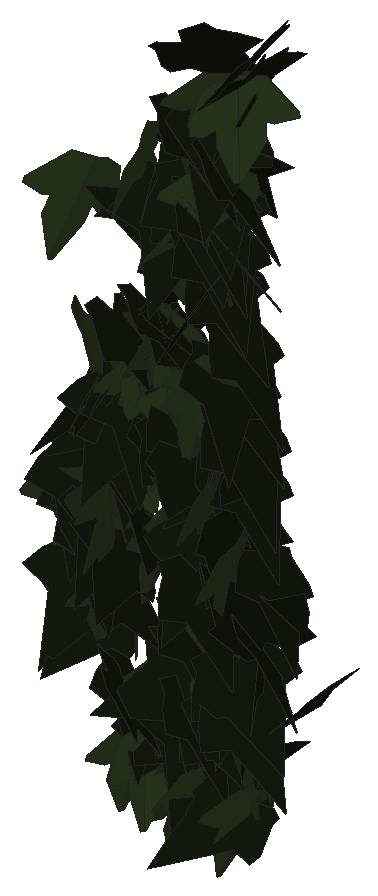
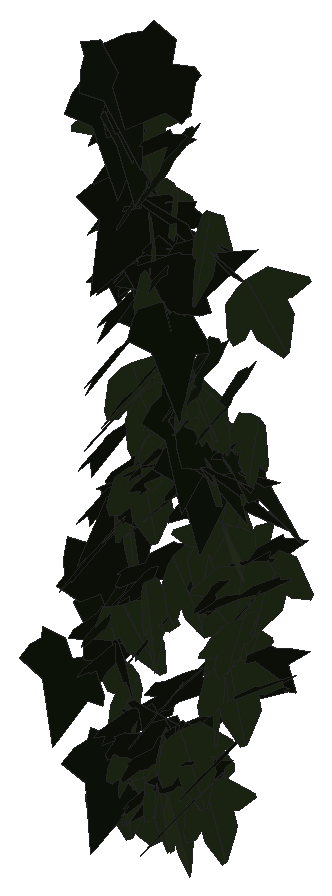
# SketchUp Ruby script. Lengths in inches.
U = 1.inch
M = Sketchup.active_model
def pt(a) = Geom::Point3d.new(a.map { |v| v * U })
def face(e, loops, mat)
  f = e.add_face(loops[0].map { |a| pt(a) })
  loops[1..].each { |l| e.add_face(l.map { |a| pt(a) }).erase! }
  f.material = f.back_material = mat if mat
  f
end
# faces: each face lists its corners as indices into pts; further lists are holes
def faces(e, pts, list, mat = nil) = list.each { |f| face(e, (f[0].is_a?(Array) ? f : [f]).map { |l| l.map { |i| pts[i] } }, mat) }
# xy, xz, yz: faces in a plane at the given z, y or x. An outline is a flat list of corners, or four numbers for a rectangle; further outlines are holes
def ring(l) = l.size == 4 ? [[l[0], l[1]], [l[2], l[1]], [l[2], l[3]], [l[0], l[3]]] : l.each_slice(2).to_a
def flat(e, list, mat, &to3) = list.each { |f| face(e, (f[0].is_a?(Array) ? f : [f]).map { |l| ring(l).map { |u, v| to3.(u, v) } }, mat) }
def xy(e, z, list, mat = nil) = flat(e, list, mat) { |x, y| [x, y, z] }
def xz(e, y, list, mat = nil) = flat(e, list, mat) { |x, z| [x, y, z] }
def yz(e, x, list, mat = nil) = flat(e, list, mat) { |y, z| [x, y, z] }
def lines(e, pts, list) = list.each { |a, b| e.add_line(pt(pts[a]), pt(pts[b])) }
# prism: a flat outline (further loops are holes) pulled along v
def prism(e, loops, v, mat = nil)
  f = face(e, loops, mat); d = Geom::Vector3d.new(v.map { |x| x * U })
  f.pushpull(f.normal.samedirection?(d) ? d.length : -d.length)
end
def box(e, o, s, mat = nil) = prism(e, [[o, [o[0] + s[0], o[1], o[2]], [o[0] + s[0], o[1] + s[1], o[2]], [o[0], o[1] + s[1], o[2]]]], [0, 0, s[2]], mat)
def at(x, y, z, deg = 0) = Geom::Transformation.translation(pt([x, y, z])) * Geom::Transformation.rotation(ORIGIN, Z_AXIS, deg.degrees)
def axes(o, x, y, z) = Geom::Transformation.new([*x, 0, *y, 0, *z, 0, *pt(o).to_a, 1])
def part(name) = M.definitions.add(name)
# library, detail: a bought-in or finely detailed component or shape, given as its bounding box
def library(name, o, s) = part(name).tap { |d| box(d.entities, o, s) }
def detail(e, o, s) = box(e.add_group.entities, o, s)
def put(e, d, t, mat = nil) = e.add_instance(d, t).tap { |i| i.material = mat if mat }
def group(e, t, mat = nil) = e.add_group.tap { |g| g.transformation = t; g.material = mat if mat }.entities
root = M.entities
M.materials.add("efeu1").color = [18, 25, 13]
M.materials.add("efeu2").color = [43, 57, 29]
c1 = part("ivyleaf_10")
p = [[0,0.5,-0.03],[-0.0625,2.02,-0.43],[-0.19,2.01,-0.46],[-0.54,1.05,-0.29],[-0.52,0.625,-0.18],[-0.83,0.76,-0.28],
  [-1.16,0.64,-0.33],[-1.15,0.33,-0.24],[-0.77,-0.39,0.02],[-0.3,-0.51,0.16],[0.04,-0.48,0.23],[-0.02,2.01,-0.4375],
  [-0.06,2.01,-0.43],[0.04,-0.49,0.23],[0.67,-0.49,0.14],[1.38,0.36,-0.2],[1.375,0.51,-0.24],[0.81,0.65,-0.19],
  [0.62,0.59,-0.15],[0.6,1.09,-0.28],[0.5,1.23,-0.31]]
faces(c1.entities,p,[[0,1,2,3,4,5,6,7,8,9,10],[11,12,0,13,14,15,16,17,18,19,20]],"efeu2")
c2 = part("ivyleaf_9")
p = [[1.54,2.16,1.25],[1.36,2.04,1.19],[-0.21,0.99,0.68],[-0.71,1.11,0.82],[-0.85,0.86,0.67],[-0.8,0.17,0.21],
  [-0.9,-0.01,0.1],[-0.67,-0.16,-0.02],[-0.08,-0.08,-0.05],[-0.03,-0.6,-0.4],[0.65,-0.88,-0.66],[0.83,-0.6,-0.49],
  [1.29,-0.42,-0.43],[1.8125,-0.07,-0.26],[1.21,0.44,0.15]]
faces(c2.entities,p,[[0,1,2,3,4,5,6,7,8,9,10,11,12,13,14]],"efeu1")
put(root,c1,axes([515.29,133.45,212.8],[-0.80305,-0.32335,-0.1119],[0.10212,0.04596,-0.8657],[0.32657,-0.80951,-0.00446]))
put(root,c2,axes([515.36,134.21,210.39],[-0.48603,-0.68308,0.11872],[-0.0493,-0.11057,-0.83801],[0.69156,-0.48795,0.0237]))
put(root,c1,axes([515.48,134.64,210.09],[-0.50146,-0.66753,0.15686],[-0.03057,-0.17238,-0.83128],[0.68503,-0.49635,0.07774]))
put(root,c2,axes([515.47,134.48,209.53],[-0.48983,-0.60352,0.33809],[-0.01133,-0.40721,-0.74332],[0.69167,-0.43407,0.22725]))
put(root,c1,axes([515.59,133.73,216.51],[-0.77942,0.38853,0.11578],[-0.12296,0.01252,-0.86982],[-0.38632,-0.78787,0.04327]))
put(root,c1,axes([515.375,134.55,211.5],[0.04627,0.85295,0.0692],[0.00684,0.06893,-0.8542],[-0.85573,0.04668,-0.00308]))
put(root,c1,axes([515.65,133.52,220.26],[-0.36653,-0.77477,0.4371],[-0.01066,-0.46889,-0.84006],[0.8895,-0.32487,0.17005]))
put(root,c2,axes([515.51,133.89,213.1],[-0.20454,-0.85126,0.02522],[-0.02053,-0.021,-0.87536],[0.85138,-0.20501,-0.01505]))
put(root,c2,axes([515.38,134.375,212.44],[-0.17335,-0.84195,-0.0494],[0.19386,0.0093,-0.83887],[0.82082,-0.18001,0.18769]))
put(root,c1,axes([515.53,134.25,212.82],[0.47061,0.7276,0.02766],[0.02328,0.01788,-0.86647],[-0.72775,0.47108,-0.00984]))
put(root,c2,axes([516.15,133.43,215.49],[-0.68936,0.51075,-0.19193],[0.10035,-0.1853,-0.85353],[-0.53631,-0.69117,0.087]))
put(root,c2,axes([515.67,134.29,212.7],[-0.0531,-0.86174,-0.09082],[-0.00711,0.09142,-0.86328],[0.86648,-0.05206,-0.01265]))
put(root,c1,axes([515.81,134.27,213.91],[0.46626,-0.59261,0.43719],[0.25158,-0.35815,-0.75376],[0.69212,0.5294,-0.02054]))
put(root,c1,axes([516.09,133.84,211.84],[-0.38547,-0.74939,0.19121],[0.03336,-0.22955,-0.83242],[0.77268,-0.36394,0.13133]))
put(root,c1,axes([516.12,133.97,210.58],[-0.15472,-0.8501,0.0923],[0.00598,-0.09487,-0.86376],[0.85507,-0.15316,0.02274]))
put(root,c2,axes([515.68,133.78,211.75],[0.20571,-0.83275,0.17944],[0.05578,-0.17104,-0.85769],[0.85004,0.21275,0.01286]))
put(root,c1,axes([516.22,134.57,206.42],[-0.24298,-0.78326,0.17958],[0.02267,-0.19422,-0.81642],[0.80326,-0.23145,0.07737]))
put(root,c2,axes([516.02,134.07,212.05],[-0.16234,-0.77343,0.35448],[-0.08781,-0.34372,-0.79016],[0.84625,-0.18403,-0.01399]))
put(root,c2,axes([516.62,134.21,215.09],[-0.84849,-0.07755,0.17646],[-0.16949,-0.07912,-0.84976],[0.09178,-0.86302,0.06205]))
put(root,c1,axes([516.28,134.3,209.93],[0.59117,-0.52975,-0.34968],[-0.08315,0.40909,-0.76035],[0.62928,0.55173,0.22802]))
put(root,c1,axes([516.12,133.52,212.74],[-0.16495,-0.8864,0.06493],[0.05275,0.05616,0.90066],[-0.88721,0.16814,0.04148]))
put(root,c1,axes([516.35,133.73,213.03],[-0.04646,-0.86798,-0.1242],[0.02358,0.12309,-0.86906],[0.8765,-0.04932,0.0168]))
put(root,c2,axes([515.96,134.84,207.62],[0.08172,-0.80698,0.22827],[0.0599,-0.22315,-0.81032],[0.83651,0.09481,0.03572]))
put(root,c1,axes([516.02,134.27,213.74],[0.56721,0.5549,0.35523],[0.20443,0.29737,-0.79095],[-0.62634,0.59956,0.06353]))
put(root,c1,axes([516.64,134.98,207.98],[-0.2977,-0.75396,0.19789],[-0.04916,-0.19325,-0.81024],[0.77795,-0.30073,0.02453]))
put(root,c2,axes([516.1,133.67,210.76],[0.57004,-0.55363,-0.32653],[-0.08496,0.36772,-0.77178],[0.63711,0.54438,0.18924]))
put(root,c2,axes([516.54,134.05,214.97],[-0.59831,-0.64533,0.00139],[0.09856,-0.09325,-0.8695],[0.63776,-0.591,0.13567]))
put(root,c2,axes([516.76,134.01,215.67],[0.11074,0.8712,0.03362],[-0.04947,0.04011,-0.87654],[-0.87044,0.10856,0.0541]))
put(root,c1,axes([516.6,132.95,212.625],[0.25317,-0.7476,-0.35306],[0.03552,0.37874,-0.77649],[0.82601,0.21285,0.1416]))
put(root,c2,axes([517.07,133.92,216.2],[-0.46371,0.74719,-0.10557],[-0.03048,-0.14235,-0.87365],[-0.754,-0.45377,0.10024]))
put(root,c2,axes([516.42,133.8,211.54],[-0.11313,-0.71017,0.49254],[0.07603,-0.50299,-0.70778],[0.8609,-0.0489,0.12723]))
put(root,c2,axes([516.32,135.09,206.64],[0.45394,-0.64181,-0.28018],[-0.04513,0.30638,-0.77497],[0.69885,0.43668,0.13194]))
put(root,c2,axes([516.58,134.11,214.71],[-0.25694,-0.83225,-0.11632],[0.01361,0.1175,-0.87074],[0.84023,-0.2564,-0.02147]))
put(root,c1,axes([516.77,134.14,215.33],[0.68092,-0.5423,-0.10008],[0.00844,0.16925,-0.85968],[0.55139,0.6671,0.13676]))
put(root,c1,axes([516.88,135.11,206.14],[0.22275,-0.79275,0.05545],[0.00747,-0.05549,-0.82341],[0.79465,0.22274,-0.0078]))
put(root,c2,axes([516.45,133.54,217.14],[0.55026,-0.69072,-0.10987],[-0.01035,0.13173,-0.88005],[0.69932,0.54544,0.07342]))
put(root,c1,axes([517.03,133.93,215.96],[-0.28301,-0.82945,0.11986],[0.01356,-0.13103,-0.87469],[0.83795,-0.27801,0.05464]))
put(root,c2,axes([516.78,134.05,215.3125],[-0.10439,-0.87209,-0.07403],[-0.00089,0.07466,-0.87827],[0.87523,-0.10394,-0.00972]))
put(root,c1,axes([516.92,133.97,206.73],[0.27693,0.80701,-0.11706],[-0.03925,-0.11029,-0.8532],[-0.81451,0.2797,0.00132]))
put(root,c2,axes([516.84,132.89,208.9],[0.73763,-0.27403,-0.46755],[-0.41717,0.21694,-0.7853],[0.34592,0.84596,0.04993]))
put(root,c2,axes([516.68,134.62,207.18],[0.25042,-0.57612,-0.54841],[0.09373,0.59232,-0.57945],[0.78987,0.11237,0.24263]))
put(root,c2,axes([517.35,133.84,216.47],[0.05893,0.86877,0.1688],[-0.02305,0.17062,-0.87011],[-0.88472,0.05342,0.03392]))
put(root,c1,axes([516.98,134.03,216.87],[-0.81277,-0.06604,-0.34802],[0.3473,0.02289,-0.81543],[0.06973,-0.88385,0.00488]))
put(root,c1,axes([517.23,133.76,216.83],[0.64335,-0.61121,-0.06337],[-0.03909,0.05086,-0.88734],[0.61324,0.64446,0.00993]))
put(root,c1,axes([517.09,133.74,216.06],[0.10849,0.81259,0.30422],[0.00524,0.30597,-0.81913],[-0.86765,0.10345,0.03309]))
put(root,c1,axes([517.28,133.27,221.38],[0.11171,-0.75215,-0.48219],[0.04222,0.48985,-0.75431],[0.89244,0.07097,0.09604]))
put(root,c1,axes([517.36,133.89,216.82],[0.09028,-0.88256,-0.05683],[-0.00008,0.05711,-0.88715],[0.88439,0.0901,0.00572]))
put(root,c1,axes([517.38,135.04,206.71],[0.01897,-0.82787,-0.03557],[0.001,0.0356,-0.82808],[0.82863,0.01891,0.00182]))
put(root,c1,axes([517.39,134.21,212.22],[0.07246,-0.88468,0.28141],[0.04261,-0.2788,-0.88744],[0.92738,0.08193,0.01878]))
put(root,c1,axes([518.02,133.34,215.7],[-0.1355,0.04894,0.8868],[-0.88801,-0.02342,-0.1344],[0.01579,-0.89678,0.0519]))
put(root,c2,axes([517.03,133.81,212.44],[0.04072,-0.56712,0.6413],[0.23385,-0.61024,-0.5545],[0.82354,0.20132,0.12575]))
put(root,c1,axes([517.51,133.84,217.11],[-0.51025,0.72885,0.03261],[-0.08067,-0.01682,-0.88648],[-0.7251,-0.51101,0.07568]))
put(root,c1,axes([517.54,134.57,207.53],[0.20361,-0.72912,-0.36426],[0.06412,0.38862,-0.74203],[0.81252,0.15204,0.14984]))
put(root,c2,axes([518.02,134.26,208.63],[-0.55301,-0.29719,0.58866],[-0.37205,-0.49369,-0.59876],[0.54445,-0.63923,0.18875]))
put(root,c2,axes([517.18,133.76,217.55],[0.55765,-0.68675,0.12788],[0.15763,-0.0357,-0.8791],[0.68053,0.57101,0.09883]))
put(root,c2,axes([518.4,133.73,219.6],[-0.08013,-0.00309,0.89127],[-0.88737,-0.08346,-0.08007],[0.0834,-0.89097,0.00441]))
put(root,c2,axes([517.43,133.69,214.77],[0.6087,-0.52528,-0.38295],[-0.10914,0.43459,-0.76961],[0.64082,0.57297,0.23267]))
put(root,c2,axes([518.17,133.69,218.83],[-0.12584,0.88894,0.02665],[-0.00201,0.02663,-0.8978],[-0.88933,-0.12584,-0.00174]))
put(root,c2,axes([517.59,134.66,206.68],[0.41321,-0.65407,-0.35834],[-0.02382,0.39788,-0.75371],[0.74542,0.37529,0.17455]))
put(root,c2,axes([518.52,134.36,207.91],[-0.82548,0.08718,0.2087],[-0.2107,-0.00937,-0.82951],[-0.0822,-0.8514,0.0305]))
put(root,c2,axes([517.84,134.71,207.41],[-0.17681,-0.86487,0.23013],[-0.03363,-0.22799,-0.88267],[0.89433,-0.17956,0.0123]))
put(root,c1,axes([518.08,134.58,211.39],[0.24976,-0.79859,-0.19078],[-0.02701,0.19131,-0.83617],[0.82061,0.24935,0.03054]))
put(root,c2,axes([517.57,133.99,217.15],[0.52021,-0.71243,-0.06599],[0.00371,0.08428,-0.88058],[0.71547,0.51757,0.05255]))
put(root,c1,axes([518.12,133.82,206.36],[0.16879,-0.82107,0.0643],[0.00909,-0.06378,-0.83823],[0.82354,0.16899,-0.00393]))
put(root,c2,axes([518.04,134.84,207.77],[-0.3887,-0.7385,-0.0891],[0.03221,0.08373,-0.83449],[0.74316,-0.38989,-0.01044]))
put(root,c2,axes([518.76,133.38,221.22],[-0.81525,0.2185,0.32741],[-0.32441,0.0535,-0.84349],[-0.22293,-0.87691,0.03012]))
put(root,c1,axes([518.21,133.85,215.45],[-0.25263,-0.70248,0.58259],[0.08392,-0.61982,-0.71098],[0.90876,-0.13805,0.22761]))
put(root,c2,axes([518.2,133.67,220.52],[-0.46727,-0.7686,-0.07696],[0.02106,0.07724,-0.89922],[0.77215,-0.46722,-0.02205]))
put(root,c2,axes([517.98,133.74,214.92],[0.22146,-0.7594,-0.41202],[-0.03742,0.41651,-0.78779],[0.86316,0.2129,0.07156]))
put(root,c1,axes([518.47,133.58,219.77],[-0.22849,-0.87335,-0.01684],[0.01555,0.01334,-0.90267],[0.87337,-0.22872,0.01166]))
put(root,c1,axes([518.5,134.31,214.45],[-0.58365,-0.6183,0.17544],[0.02028,-0.25459,-0.82975],[0.64239,-0.55372,0.1856]))
put(root,c2,axes([518.02,134.14,208.27],[0.36561,-0.76695,-0.06637],[-0.02591,0.06118,-0.84963],[0.76938,0.36652,0.00293]))
put(root,c1,axes([518.52,133.77,206.62],[-0.17419,-0.8244,-0.0312],[0.00419,0.031,-0.84259],[0.82498,-0.17422,-0.00231]))
put(root,c2,axes([518.08,133.83,215.42],[0.24519,-0.82456,-0.192],[-0.01027,0.19698,-0.85905],[0.84655,0.2412,0.04519]))
put(root,c1,axes([518.63,134.5,205.05],[0.79976,0.09118,0.33671],[-0.3339,-0.04369,0.80492],[0.10098,-0.86665,-0.00516]))
put(root,c2,axes([518.51,134.125,212.1],[-0.37665,-0.75517,0.19103],[-0.02257,-0.20152,-0.84114],[0.77863,-0.37114,0.06803]))
put(root,c1,axes([518.67,134.43,206.82],[-0.19334,-0.77409,-0.25419],[0.06035,0.24693,-0.79787],[0.81252,-0.20254,-0.00123]))
put(root,c2,axes([518.28,133.81,210.39],[0.31497,-0.82423,-0.04069],[-0.00841,0.04034,-0.88234],[0.82519,0.31502,0.00654]))
put(root,c1,axes([518.78,133.125,221.65],[-0.76435,0.4883,0.06405],[-0.0507,0.03961,-0.90699],[-0.48987,-0.766,-0.00607]))
put(root,c1,axes([518.89,134.73,206.35],[-0.53594,-0.62148,0.1296],[-0.05013,-0.12765,-0.81943],[0.63287,-0.53641,0.04485]))
put(root,c1,axes([518.79,133.78,216.1],[-0.113,-0.81754,0.31871],[0.0879,-0.33027,-0.81603],[0.87305,-0.07256,0.12341]))
put(root,c2,axes([518.95,134.68,206.66],[0.27329,0.79502,0.12704],[-0.00227,0.13492,-0.83945],[-0.8051,0.26949,0.04549]))
put(root,c2,axes([518.54,133.12,214.79],[0.44089,-0.58927,-0.48643],[-0.15002,0.48391,-0.72219],[0.74923,0.44365,0.14164]))
put(root,c2,axes([518.53,134.4,208.04],[0.18775,-0.71682,-0.39271],[0.04514,0.41141,-0.72938],[0.81609,0.14216,0.13069]))
put(root,c1,axes([519.5,133.1,219.47],[-0.35497,0.16347,0.82727],[-0.80528,0.20065,-0.38518],[-0.25025,-0.87756,0.06603]))
put(root,c2,axes([518.98,134.38,214.41],[-0.52559,-0.59521,0.34471],[-0.02108,-0.41968,-0.75681],[0.6875,-0.4679,0.24032]))
put(root,c2,axes([518.65,133.52,211.67],[0.23198,-0.81167,-0.19024],[-0.01152,0.19433,-0.84315],[0.83358,0.22856,0.04129]))
put(root,c1,axes([519.03,133.48,221.05],[0.5587,-0.67737,-0.23325],[0.02387,0.31322,-0.85247],[0.71601,0.51811,0.21042]))
put(root,c2,axes([518.54,133.21,222.85],[0.51034,-0.76669,-0.01494],[0.04373,0.04701,-0.91889],[0.76559,0.50839,0.06244]))
put(root,c1,axes([519.16,133.95,210.29],[0.74638,0.331,-0.305],[-0.30465,-0.06325,-0.81416],[-0.33132,0.80381,0.06153]))
put(root,c1,axes([519.22,133.67,216.72],[-0.42601,-0.73898,0.20711],[-0.04457,-0.21265,-0.85045],[0.76616,-0.42327,0.06569]))
put(root,c2,axes([519.14,132.28,218.23],[0.29843,0.29509,0.82603],[0.14187,0.8448,-0.35305],[-0.8656,0.2402,0.22692]))
put(root,c2,axes([519.55,134.05,206.32],[-0.73291,-0.31909,0.29154],[-0.24869,-0.15809,-0.79821],[0.35351,-0.77277,0.04291]))
put(root,c2,axes([519.06,133.6,221.77],[0.70414,0.5638,-0.04726],[-0.04198,-0.02319,-0.902],[-0.56422,0.70534,0.00813]))
put(root,c2,axes([518.91,133.52,220.98],[-0.37837,-0.47497,-0.67524],[0.39708,0.54651,-0.60693],[0.72379,-0.54812,-0.02002]))
put(root,c2,axes([519.73,133.29,222.96],[-0.11681,0.60112,0.68361],[-0.22231,0.64951,-0.60912],[-0.88275,-0.24311,0.06294]))
put(root,c2,axes([519.01,133.37,221.33],[-0.25256,-0.77284,-0.39845],[0.2189,0.34504,-0.808],[0.8415,-0.32171,0.0906]))
put(root,c2,axes([518.89,133.55,220.76],[0.38481,-0.81893,0.04314],[0.05003,-0.02412,-0.90416],[0.81854,0.38646,0.03499]))
put(root,c1,axes([519.48,132.84,214.35],[0.10001,-0.78517,-0.42269],[-0.05637,0.41892,-0.79151],[0.88993,0.11478,-0.00263]))
put(root,c2,axes([518.75,133.44,220.37],[0.7574,-0.43331,0.22126],[0.19429,-0.10596,-0.87257],[0.44605,0.78191,0.00437]))
put(root,c1,axes([519.5,133.24,221.46],[-0.51766,-0.70405,0.23317],[0.01287,-0.29283,-0.85563],[0.74155,-0.4864,0.17762]))
put(root,c1,axes([519.59,133.22,223.87],[-0.44905,-0.78383,0.16258],[-0.07611,-0.14377,-0.90333],[0.79689,-0.45543,0.00534]))
put(root,c2,axes([519.13,132.58,225.04],[0.78654,0.45963,0.17256],[0.14076,0.10108,-0.91085],[-0.47034,0.79888,0.01597]))
put(root,c2,axes([519.15,133.8,216.59],[0.13608,-0.85215,0.19138],[0.02471,-0.18986,-0.86293],[0.87303,0.1382,-0.00541]))
put(root,c1,axes([519.64,134.03,206.28],[-0.10651,-0.79215,0.30213],[-0.04685,-0.29854,-0.79925],[0.84651,-0.1162,-0.00622]))
put(root,c2,axes([519.09,134.25,216.3125],[0.38679,-0.7726,-0.13519],[0.00889,0.15505,-0.86062],[0.78429,0.37927,0.07643]))
put(root,c2,axes([519.4,133.52,222.89],[-0.2538,-0.87101,-0.03018],[-0.00072,0.03164,-0.90718],[0.87153,-0.25362,-0.00953]))
put(root,c2,axes([519.24,133.51,220.05],[0.14222,-0.86709,-0.16141],[0.01945,0.16654,-0.8775],[0.88177,0.13618,0.04539]))
put(root,c2,axes([519.61,133.21,213.66],[0.18204,-0.07427,-0.86937],[-0.48005,0.73307,-0.16315],[0.72861,0.50155,0.10972]))
put(root,c1,axes([519.52,133.63,208.04],[-0.72297,0.49216,-0.18339],[0.147,-0.10994,-0.87456],[-0.50423,-0.73772,0.00799]))
put(root,c2,axes([519.26,133.5,219.19],[0.33008,-0.79042,-0.25721],[-0.02095,0.26875,-0.85276],[0.83095,0.32075,0.08068]))
put(root,c2,axes([519.3,134.37,214.11],[0.25347,-0.82244,-0.09754],[-0.00147,0.10156,-0.86015],[0.82821,0.25188,0.02833]))
put(root,c2,axes([519.51,134.16,209.58],[-0.44014,0.03671,-0.72642],[0.72147,-0.08569,-0.44147],[-0.09228,-0.84502,0.01322]))
put(root,c2,axes([519.34,133.28,222.14],[0.66742,-0.61661,-0.10554],[-0.06567,0.08441,-0.90849],[0.62212,0.67042,0.01732]))
put(root,c1,axes([519.91,133.09,212.76],[0.11795,-0.87056,-0.15486],[-0.0028,0.15586,-0.87833],[0.88422,0.11663,0.01787]))
put(root,c2,axes([520.12,133.27,224.25],[0.06279,0.91278,-0.01474],[-0.05683,-0.01084,-0.91322],[-0.91112,0.06358,0.05594]))
put(root,c2,axes([519.49,133.93,215.4375],[0.28388,-0.89558,-0.14098],[-0.0258,0.13969,-0.93933],[0.90624,0.28452,0.01742]))
put(root,c2,axes([519.53,133.84,217.66],[0.37477,-0.79034,-0.14379],[-0.03345,0.14317,-0.87415],[0.80261,0.37501,0.03071]))
put(root,c2,axes([520.2,133.8,210.6],[0.46952,0.00828,0.71979],[-0.71769,-0.06104,0.46885],[0.05564,-0.85722,-0.02643]))
put(root,c2,axes([520.41,133.04,224.9],[-0.27151,0.88535,-0.03982],[-0.0142,-0.04598,-0.92565],[-0.88613,-0.27053,0.02703]))
put(root,c2,axes([519.76,133.6,209.93],[-0.03045,-0.7035,-0.54291],[0.02566,0.54231,-0.70415],[0.88826,-0.03978,0.00173]))
put(root,c1,axes([519.97,133.22,223.73],[0.6167,0.68403,0.02259],[-0.06349,0.08746,-0.91491],[-0.68145,0.61089,0.10569]))
put(root,c2,axes([519.76,133.51,209.09],[0.22266,-0.78651,-0.31242],[0.02897,0.32995,-0.80998],[0.84579,0.19575,0.11]))
put(root,c2,axes([519.94,134.39,212.05],[0.27144,-0.81931,0.02453],[0.00634,-0.02374,-0.8631],[0.81965,0.27151,-0.00145]))
put(root,c2,axes([519.79,133.98,210.44],[0.44172,-0.65348,0.37756],[0.2025,-0.31881,-0.7887],[0.72703,0.48583,-0.00972]))
put(root,c2,axes([520.66,134.44,208.73],[0.12529,0.79836,0.29937],[-0.08578,0.31285,-0.79841],[-0.84831,0.08628,0.12495]))
